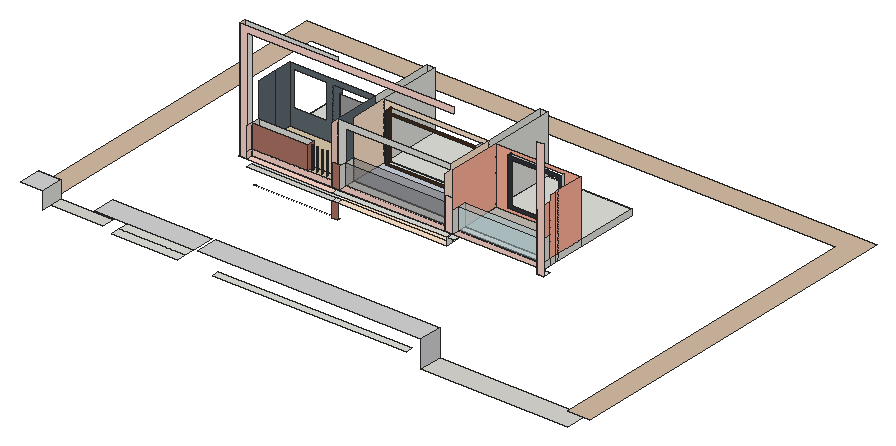
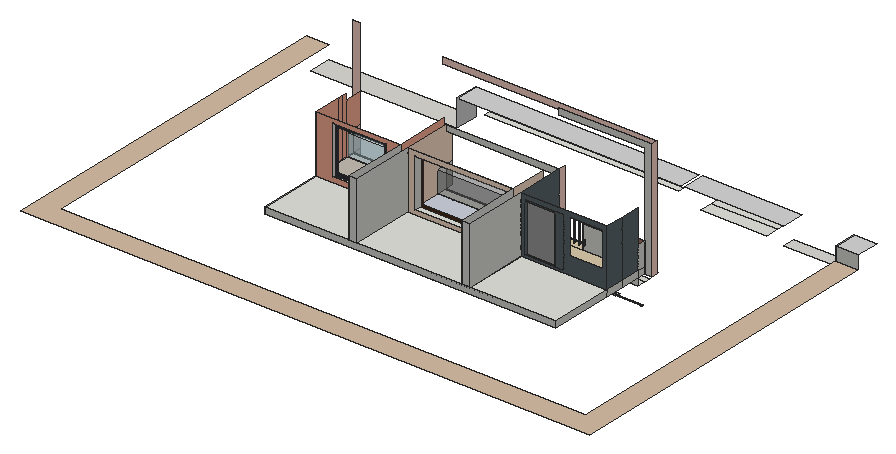
# SketchUp Ruby script. Lengths in inches.
U = 1.inch
M = Sketchup.active_model
def pt(a) = Geom::Point3d.new(a.map { |v| v * U })
def face(e, loops, mat)
  f = e.add_face(loops[0].map { |a| pt(a) })
  loops[1..].each { |l| e.add_face(l.map { |a| pt(a) }).erase! }
  f.material = f.back_material = mat if mat
  f
end
# faces: each face lists its corners as indices into pts; further lists are holes
def faces(e, pts, list, mat = nil) = list.each { |f| face(e, (f[0].is_a?(Array) ? f : [f]).map { |l| l.map { |i| pts[i] } }, mat) }
# xy, xz, yz: faces in a plane at the given z, y or x. An outline is a flat list of corners, or four numbers for a rectangle; further outlines are holes
def ring(l) = l.size == 4 ? [[l[0], l[1]], [l[2], l[1]], [l[2], l[3]], [l[0], l[3]]] : l.each_slice(2).to_a
def flat(e, list, mat, &to3) = list.each { |f| face(e, (f[0].is_a?(Array) ? f : [f]).map { |l| ring(l).map { |u, v| to3.(u, v) } }, mat) }
def xy(e, z, list, mat = nil) = flat(e, list, mat) { |x, y| [x, y, z] }
def xz(e, y, list, mat = nil) = flat(e, list, mat) { |x, z| [x, y, z] }
def yz(e, x, list, mat = nil) = flat(e, list, mat) { |y, z| [x, y, z] }
def lines(e, pts, list) = list.each { |a, b| e.add_line(pt(pts[a]), pt(pts[b])) }
# prism: a flat outline (further loops are holes) pulled along v
def prism(e, loops, v, mat = nil)
  f = face(e, loops, mat); d = Geom::Vector3d.new(v.map { |x| x * U })
  f.pushpull(f.normal.samedirection?(d) ? d.length : -d.length)
end
def box(e, o, s, mat = nil) = prism(e, [[o, [o[0] + s[0], o[1], o[2]], [o[0] + s[0], o[1] + s[1], o[2]], [o[0], o[1] + s[1], o[2]]]], [0, 0, s[2]], mat)
def at(x, y, z, deg = 0) = Geom::Transformation.translation(pt([x, y, z])) * Geom::Transformation.rotation(ORIGIN, Z_AXIS, deg.degrees)
def axes(o, x, y, z) = Geom::Transformation.new([*x, 0, *y, 0, *z, 0, *pt(o).to_a, 1])
def part(name) = M.definitions.add(name)
# library, detail: a bought-in or finely detailed component or shape, given as its bounding box
def library(name, o, s) = part(name).tap { |d| box(d.entities, o, s) }
def detail(e, o, s) = box(e.add_group.entities, o, s)
def put(e, d, t, mat = nil) = e.add_instance(d, t).tap { |i| i.material = mat if mat }
def group(e, t, mat = nil) = e.add_group.tap { |g| g.transformation = t; g.material = mat if mat }.entities
root = M.entities
M.materials.add("[Blinds Vertical Pattern]").color = [212, 212, 214]
M.materials.add("[Blinds Vertical Stripe Gray]").color = [160, 160, 160]
M.materials.add("[Color B01]").color = [255, 216, 204]
M.materials.add("[Color B02]").color = [255, 178, 153]
M.materials.add("[Color C01]").color = [255, 229, 204]
M.materials.add("[Field Rectangle Tile]").color = [196, 189, 179]
M.materials.add("[Field Square Tile]").color = [217, 201, 169]
M.materials.add("[Formica Graystone]").color = [149, 146, 135]
M.materials.add("[Formica Laminate Dark]").color = [50, 53, 60]
M.materials.add("[Formica Laminate Light]").color = [213, 189, 164]
M.materials.add("[Formica Speckled Grey]").color = [94, 105, 111]
M.materials.add("[Marble Carrara Floor Tile]").color = [204, 208, 219]
M.materials.add("[Stone Flagstone Ashlar]").color = [175, 116, 102]
M.materials.add("[Stone Flagstone Ashlar]1").color = [175, 116, 102]
M.materials.add("[Terrazzo Tile Light]").color = [219, 217, 210]
M.materials.add("[Translucent Glass Gray]").color = [128, 128, 128]
M.materials["[Translucent Glass Gray]"].alpha = 0.5
M.materials.add("[Translucent Glass Safety]").color = [204, 235, 244]
M.materials["[Translucent Glass Safety]"].alpha = 0.5
M.materials.add("[Wood Veneer 01]").color = [76, 44, 23]
xy(root,546.8125,[[2439.95,0,3329.24,137.64]],"[Terrazzo Tile Light]")
xy(root,604.375,[[137.64,62.625,453.55,137.64]],"[Terrazzo Tile Light]")
xy(root,610.51,[[1170.21,0,2349.69,42.1875]])
xy(root,619.23,[[1302.08,955.61,1426.75,983.36],[1442.97,955.61,1568.8125,983.36],[1585.03,955.61,1721.6875,983.36],[1737.9,955.61,1860.8,983.36]])
xy(root,623.51,[[554.87,0,956.3,58.3125],[554.87,58.3125,956.3,137.64]])
xy(root,631.3125,[[3329.24,0,3466.875,0,3466.875,2178.1875,0,2178.1875,0,137.64,137.64,137.64,137.64,2040.55,3329.24,2040.55]],"[Formica Laminate Light]")
xy(root,636.3125,[[1285,955.61,1877.875,983.36]],"[Wood Veneer 01]")
xy(root,642.77,[[914.91,1040.67,1175.1,1074.11]])
xy(root,646.07,[[723.26,1062.73,783.24,1074.11],[797.04,1062.73,861.24,1074.11]],"[Formica Speckled Grey]")
xy(root,657.36,[[1213.16,856.3125,1248.61,894.5]])
xy(root,657.36,[[1248.61,856.3125,1908.08,894.5],[1248.61,894.5,1908.08,950.43]],"[Color C01]")
xy(root,657.36,[[691.11,856.3125,1213.16,894.5],[691.11,894.5,1213.16,950.43]],"[Terrazzo Tile Light]")
xy(root,659.05,[[710.28,1062.73,874.22,1074.11]])
xy(root,659.56,[[2059.65,990.79,2174.84,1012.29],[2197.86,990.79,2308.19,1012.29]])
xy(root,672.85,[[2046.36,990.79,2321.48,1012.29]],"[Formica Laminate Dark]")
xy(root,702.75,[[2463.34,849.3125,2507.95,856.3125],[1213.16,856.3125,1908.08,894.5],[1908.08,856.3125,1953.74,899.87],[2463.34,856.3125,2507.95,894.5],[646.49,861.43,691.11,894.5],
  [646.49,894.5,691.11,899.87],[691.11,894.5,1213.16,899.87],[1213.16,894.5,1248.61,899.87],[1248.61,894.5,1908.08,899.87],[691.11,899.87,1213.16,950.43],
  [1213.16,899.87,1248.61,1126.61],[1248.61,899.87,1908.08,950.43],[1908.08,899.87,1938.3,1126.61],[1938.3,899.87,1953.74,1012.29],[691.11,950.43,1213.16,1074.11],
  [1248.61,950.43,1908.08,983.36],[1248.61,983.36,1248.61,1126.61,1213.16,1126.61,1213.16,1074.11,691.11,1074.11,691.11,1182.72,2463.34,1182.72,2463.34,1012.29,1938.3,1012.29,1938.3,1126.61,1908.08,1126.61,1908.08,983.36],[691.11,1182.72,2463.34,1571.68]])
xy(root,702.75,[[646.49,856.3125,1213.16,856.3125,1213.16,894.5,691.11,894.5,691.11,861.43,646.49,861.43]],"[Color B01]")
xy(root,702.75,[[1953.74,899.87,2463.34,1012.29]],"[Color B02]")
xy(root,712.1875,[[0,0,137.64,137.64],[453.55,0,1057.62,137.64],[1080.95,0,2439.95,137.64]],"[Blinds Vertical Pattern]")
xy(root,738.75,[[1214.63,849.3125,1263.92,894.5],[1905.54,849.3125,1950.59,899.87],[1214.63,894.5,1263.92,899.87],[1263.92,894.5,1905.54,899.87],[1950.59,894.5,2463.34,899.87],
  [691.11,899.87,1027.33,950.43],[1214.63,899.87,1263.92,1571.68],[1263.92,899.87,1905.54,954.56],[1905.54,899.87,1950.59,1571.68],[1950.59,899.87,2463.34,942.43],
  [1041.89,916.51,1040.81,916.65,1039.8,917.07,1038.93,917.73,1038.27,918.6,1037.85,919.61,1037.71,920.69,1037.85,921.78,1038.27,922.79,1038.93,923.65,1039.8,924.32,1040.81,924.74,1041.89,924.88,1042.98,924.74,1043.99,924.32,1044.85,923.65,1045.52,922.79,1045.9375,921.78,1046.08,920.69,1045.9375,919.61,1045.52,918.6,1044.85,917.73,1043.99,917.07,1042.98,916.65],[1070.77,916.51,1069.68,916.65,1068.67,917.07,1067.81,917.73,1067.14,918.6,1066.72,919.61,1066.58,920.69,1066.72,921.78,1067.14,922.79,1067.81,923.65,1068.67,924.32,1069.68,924.74,1070.77,924.88,1071.85,924.74,1072.86,924.32,1073.73,923.65,1074.39,922.79,1074.8125,921.78,1074.96,920.69,1074.8125,919.61,1074.39,918.6,1073.73,917.73,1072.86,917.07,1071.85,916.65],[1101.58,916.51,1100.5,916.65,1099.49,917.07,1098.62,917.73,1097.95,918.6,1097.54,919.61,1097.39,920.69,1097.54,921.78,1097.95,922.79,1098.62,923.65,1099.49,924.32,1100.5,924.74,1101.58,924.88,1102.66,924.74,1103.67,924.32,1104.54,923.65,1105.21,922.79,1105.625,921.78,1105.77,920.69,1105.625,919.61,1105.21,918.6,1104.54,917.73,1103.67,917.07,1102.66,916.65],[1131.83,916.51,1130.75,916.65,1129.74,917.07,1128.87,917.73,1128.2,918.6,1127.79,919.61,1127.64,920.69,1127.79,921.78,1128.2,922.79,1128.87,923.65,1129.74,924.32,1130.75,924.74,1131.83,924.88,1132.91,924.74,1133.92,924.32,1134.79,923.65,1135.46,922.79,1135.875,921.78,1136.02,920.69,1135.875,919.61,1135.46,918.6,1134.79,917.73,1133.92,917.07,1132.91,916.65],[1167.14,916.51,1166.06,916.65,1165.05,917.07,1164.18,917.73,1163.52,918.6,1163.1,919.61,1162.96,920.69,1163.1,921.78,1163.52,922.79,1164.18,923.65,1165.05,924.32,1166.06,924.74,1167.14,924.88,1168.23,924.74,1169.24,924.32,1170.1,923.65,1170.77,922.79,1171.1875,921.78,1171.33,920.69,1171.1875,919.61,1170.77,918.6,1170.1,917.73,1169.24,917.07,1168.23,916.65],
  [1198.52,916.51,1197.43,916.65,1196.42,917.07,1195.56,917.73,1194.89,918.6,1194.47,919.61,1194.33,920.69,1194.47,921.78,1194.89,922.79,1195.56,923.65,1196.42,924.32,1197.43,924.74,1198.52,924.88,1199.6,924.74,1200.61,924.32,1201.48,923.65,1202.14,922.79,1202.5625,921.78,1202.71,920.69,1202.5625,919.61,1202.14,918.6,1201.48,917.73,1200.61,917.07,1199.6,916.65],[691.11,1182.72,1214.63,1571.68],[1263.92,1182.72,1905.54,1571.68],[1950.59,1182.72,2463.34,1571.68]])
xy(root,738.75,[[1950.59,942.43,2463.34,1182.72]],"[Field Rectangle Tile]")
xy(root,738.75,[[[1027.33,899.87,1214.63,950.43],[1041.89,916.51,1040.81,916.65,1039.8,917.07,1038.93,917.73,1038.27,918.6,1037.85,919.61,1037.71,920.69,1037.85,921.78,1038.27,922.79,1038.93,923.65,1039.8,924.32,1040.81,924.74,1041.89,924.88,1042.98,924.74,1043.99,924.32,1044.85,923.65,1045.52,922.79,1045.9375,921.78,1046.08,920.69,1045.9375,919.61,1045.52,918.6,1044.85,917.73,1043.99,917.07,1042.98,916.65],[1198.52,916.51,1197.43,916.65,1196.42,917.07,1195.56,917.73,1194.89,918.6,1194.47,919.61,1194.33,920.69,1194.47,921.78,1194.89,922.79,1195.56,923.65,1196.42,924.32,1197.43,924.74,1198.52,924.88,1199.6,924.74,1200.61,924.32,1201.48,923.65,1202.14,922.79,1202.5625,921.78,1202.71,920.69,1202.5625,919.61,1202.14,918.6,1201.48,917.73,1200.61,917.07,1199.6,916.65],[1070.77,916.51,1069.68,916.65,1068.67,917.07,1067.81,917.73,1067.14,918.6,1066.72,919.61,1066.58,920.69,1066.72,921.78,1067.14,922.79,1067.81,923.65,1068.67,924.32,1069.68,924.74,1070.77,924.88,1071.85,924.74,1072.86,924.32,1073.73,923.65,1074.39,922.79,1074.8125,921.78,1074.96,920.69,1074.8125,919.61,1074.39,918.6,1073.73,917.73,1072.86,917.07,1071.85,916.65],[1167.14,916.51,1166.06,916.65,1165.05,917.07,1164.18,917.73,1163.52,918.6,1163.1,919.61,1162.96,920.69,1163.1,921.78,1163.52,922.79,1164.18,923.65,1165.05,924.32,1166.06,924.74,1167.14,924.88,1168.23,924.74,1169.24,924.32,1170.1,923.65,1170.77,922.79,1171.1875,921.78,1171.33,920.69,1171.1875,919.61,1170.77,918.6,1170.1,917.73,1169.24,917.07,1168.23,916.65],[1101.58,916.51,1100.5,916.65,1099.49,917.07,1098.62,917.73,1097.95,918.6,1097.54,919.61,1097.39,920.69,1097.54,921.78,1097.95,922.79,1098.62,923.65,1099.49,924.32,1100.5,924.74,1101.58,924.88,1102.66,924.74,1103.67,924.32,1104.54,923.65,1105.21,922.79,1105.625,921.78,1105.77,920.69,1105.625,919.61,1105.21,918.6,1104.54,917.73,1103.67,917.07,1102.66,916.65],[1131.83,916.51,1130.75,916.65,1129.74,917.07,1128.87,917.73,1128.2,918.6,1127.79,919.61,1127.64,920.69,1127.79,921.78,1128.2,922.79,1128.87,923.65,1129.74,924.32,1130.75,924.74,1131.83,924.88,1132.91,924.74,1133.92,924.32,1134.79,923.65,1135.46,922.79,1135.875,921.78,1136.02,920.69,1135.875,919.61,1135.46,918.6,1134.79,917.73,1133.92,917.07,1132.91,916.65]],[691.11,950.43,1214.63,1182.72]],"[Field Square Tile]")
xy(root,738.75,[[1263.92,954.56,1905.54,1182.72]],"[Marble Carrara Floor Tile]")
xy(root,750.91,[[1009.02,1166.28,1195.59,1182.72]])
xy(root,762.1,[[1310.9,1141.09,1861.28,1182.72]])
xy(root,769.59,[[2036.23,1166.78,2361.3,1182.72]])
xz(root,137.64,[[0,631.3125,137.64,712.1875]])
xz(root,849.3125,[[2463.34,702.75,2507.95,1424.1875],[1905.54,738.75,1950.59,937.95]],"[Color B01]")
xz(root,849.3125,[[1214.63,738.75,1263.92,872.4]],"[Stone Flagstone Ashlar]1")
xz(root,856.3125,[[1213.16,566.24,1248.61,657.36]],"[Stone Flagstone Ashlar]1")
xz(root,861.43,[[646.49,702.75,691.11,702.75,691.11,1387.1,1950.59,1387.1,1950.59,1424.1875,646.49,1424.1875]],"[Color B01]")
xz(root,894.5,[[1214.63,738.75,1214.63,1086.8125,1905.54,1086.8125,1905.54,1051.41,1263.92,1051.41,1263.92,738.75]])
xz(root,894.5,[[1263.92,738.75,1905.54,868.4375]],"[Translucent Glass Gray]")
xz(root,894.5,[[1950.59,738.75,2463.34,868.4375]],"[Translucent Glass Safety]")
xz(root,899.87,[[646.49,702.75,646.49,1424.1875,1214.63,1424.1875,1214.63,1387.1,691.11,1387.1,691.11,702.75]])
xz(root,899.87,[[691.11,702.75,2463.34,738.75]],"[Color B01]")
xz(root,899.87,[[691.11,738.75,1027.33,880]],"[Stone Flagstone Ashlar]")
xz(root,942.43,[[1950.59,738.75,2463.34,868.4375]],"[Translucent Glass Safety]")
xz(root,950.43,[[691.11,657.36,1213.16,702.75],[1248.61,657.36,1908.08,702.75],[691.11,738.75,1027.33,880]])
xz(root,954.56,[[1263.92,738.75,1905.54,868.4375]],"[Translucent Glass Gray]")
xz(root,1141.09,[[[1310.9,762.1,1861.28,1059.16],[1324.98,776.18,1847.2,1045.08]]],"[Wood Veneer 01]")
xz(root,1166.28,[[1009.02,750.91,1195.59,1033.9]],"[Blinds Vertical Stripe Gray]")
xz(root,1166.78,[[[2036.23,769.59,2361.3,1063.34],[2056.09,789.44,2341.44,1043.49]]],"[Formica Laminate Dark]")
xz(root,1182.72,[[[1950.59,738.75,2463.34,1086.8125],[2036.23,769.59,2361.3,1063.34]]],"[Color B02]")
xz(root,1182.72,[[[1263.92,738.75,1905.54,1086.8125],[1310.9,762.1,1861.28,1059.16]]],"[Color C01]")
xz(root,1182.72,[[[691.11,738.75,1214.63,1086.8125],[955.69,750.91,955.69,1058.91,917.47,1058.91,917.47,844.43,715.78,844.43,715.78,1058.91,1195.59,1058.91,1195.59,750.91]],[955.69,750.91,1009.02,1058.91]],"[Formica Speckled Grey]")
xz(root,1571.68,[[691.11,702.75,2463.34,738.75],[1214.63,738.75,1263.92,1086.8125],[1905.54,738.75,1950.59,1086.8125]])
yz(root,137.64,[[0,604.375,137.64,712.1875]])
yz(root,646.49,[[861.43,702.75,899.87,1424.1875]],"[Color B01]")
yz(root,691.11,[[899.87,702.75,950.43,738.75],[950.43,702.75,1074.11,738.75],[1074.11,702.75,1182.72,738.75],[1182.72,702.75,1571.68,738.75],[899.87,738.75,950.43,880]])
yz(root,691.11,[[861.43,702.75,899.87,738.75],[861.43,738.75,899.87,880]],"[Color B01]")
yz(root,691.11,[[950.43,738.75,1074.11,1086.8125],[1074.11,738.75,1182.72,1086.8125]],"[Formica Speckled Grey]")
yz(root,1009.02,[[1166.28,750.91,1182.72,1033.9]],"[Formica Speckled Grey]")
yz(root,1027.33,[[[899.87,738.75,950.43,880],[922.52,862.65,921.05,862.84,919.68,863.41,918.5,864.32,917.6,865.49,917.03,866.87,916.84,868.34,917.03,869.81,917.6,871.18,918.5,872.36,919.68,873.26,921.05,873.83,922.52,874.02,923.99,873.83,925.37,873.26,926.54,872.36,927.45,871.18,928.02,869.81,928.21,868.34,928.02,866.87,927.45,865.49,926.54,864.32,925.37,863.41,923.99,862.84]]],"[Stone Flagstone Ashlar]")
yz(root,1195.59,[[1166.28,750.91,1182.72,1033.9]],"[Formica Speckled Grey]")
yz(root,1214.63,[[1182.72,738.75,1571.68,1086.8125]])
yz(root,1214.63,[[849.3125,738.75,894.5,1086.8125]],"[Color B01]")
yz(root,1214.63,[[[894.5,738.75,1182.72,1086.8125],[922.52,862.65,923.99,862.84,925.37,863.41,926.54,864.32,927.45,865.49,928.02,866.87,928.21,868.34,928.02,869.81,927.45,871.18,926.54,872.36,925.37,873.26,923.99,873.83,922.52,874.02,921.05,873.83,919.68,873.26,918.5,872.36,917.6,871.18,917.03,869.81,916.84,868.34,917.03,866.87,917.6,865.49,918.5,864.32,919.68,863.41,921.05,862.84]]],"[Formica Speckled Grey]")
yz(root,1263.92,[[849.3125,738.75,894.5,868.4375],[894.5,738.75,954.56,868.4375],[1182.72,738.75,1571.68,1086.8125]])
yz(root,1263.92,[[954.56,738.75,1182.72,1086.8125]],"[Color C01]")
yz(root,1310.9,[[1141.09,762.1,1182.72,1059.16]],"[Wood Veneer 01]")
yz(root,1861.28,[[1141.09,762.1,1182.72,1059.16]])
yz(root,1905.54,[[849.3125,738.75,894.5,868.4375],[894.5,738.75,954.56,868.4375],[1182.72,738.75,1571.68,1086.8125]])
yz(root,1905.54,[[[954.56,738.75,954.56,868.4375,849.3125,868.4375,849.3125,1051.41,894.5,1051.41,894.5,1086.8125,1182.72,1086.8125,1182.72,738.75],[923.73,877.96,925.46,878.18,927.08,878.85,928.46,879.91,929.52,881.3,930.19,882.91,930.42,884.64,930.19,886.375,929.52,887.99,928.46,889.37,927.08,890.43,925.46,891.1,923.73,891.33,922,891.1,920.39,890.43,919,889.37,917.94,887.99,917.27,886.375,917.04,884.64,917.27,882.91,917.94,881.3,919,879.91,920.39,878.85,922,878.18]]],"[Color C01]")
yz(root,1908.08,[[856.3125,657.36,894.5,702.75]])
yz(root,1950.59,[[849.3125,738.75,894.5,868.4375],[894.5,738.75,942.43,868.4375],[1182.72,738.75,1571.68,1086.8125]])
yz(root,1950.59,[[[942.43,738.75,1182.72,738.75,1182.72,1086.8125,849.3125,1086.8125,849.3125,868.4375,942.43,868.4375],[918.47,876.58,917.1875,876.75,916,877.24,914.97,878.03,914.1875,879.05,913.7,880.24,913.53,881.52,913.7,882.8,914.1875,883.99,914.97,885.01,916,885.8,917.1875,886.29,918.47,886.46,919.74,886.29,920.93,885.8,921.96,885.01,922.74,883.99,923.23,882.8,923.4,881.52,923.23,880.24,922.74,879.05,921.96,878.03,920.93,877.24,919.74,876.75]]],"[Color B02]")
yz(root,2036.23,[[1166.78,769.59,1182.72,1063.34]],"[Formica Laminate Dark]")
yz(root,2361.3,[[1166.78,769.59,1182.72,1063.34]])
yz(root,2439.95,[[0,546.8125,137.64,712.1875]],"[Blinds Vertical Pattern]")
yz(root,2463.34,[[899.87,702.75,950.43,738.75],[950.43,702.75,983.36,738.75],[983.36,702.75,1012.29,738.75],[1012.29,702.75,1182.72,738.75],[1182.72,702.75,1571.68,738.75],
  [894.5,738.75,942.43,868.4375]])
yz(root,2463.34,[[849.3125,702.75,899.87,738.75],[849.3125,738.75,894.5,868.4375]],"[Color B01]")
yz(root,2463.34,[[[942.43,738.75,942.43,868.4375,849.3125,868.4375,849.3125,1051.41,950.43,1051.41,950.43,738.75],[918.47,876.58,919.74,876.75,920.93,877.24,921.96,878.03,922.74,879.05,923.23,880.24,923.4,881.52,923.23,882.8,922.74,883.99,921.96,885.01,920.93,885.8,919.74,886.29,918.47,886.46,917.1875,886.29,916,885.8,914.97,885.01,914.1875,883.99,913.7,882.8,913.53,881.52,913.7,880.24,914.1875,879.05,914.97,878.03,916,877.24,917.1875,876.75]],[950.43,738.75,950.43,1051.41,954.56,1051.41,954.56,1086.8125,983.36,1086.8125,983.36,738.75],[983.36,738.75,1012.29,1086.8125],[1012.29,738.75,1182.72,1086.8125]],"[Color B02]")
p = [[1213.16,911.02,535.46],[1213.16,911.77,536.03],[691.11,911.77,536.03],[691.11,911.02,535.46],[1213.16,915.37,536.03],[1213.16,916.11,535.46],
  [691.11,916.11,535.46],[691.11,915.37,536.03],[1213.16,912.64,536.39],[691.11,912.64,536.39],[1213.16,914.5,536.39],[691.11,914.5,536.39],
  [1213.16,913.57,536.52],[691.11,913.57,536.52],[1040.81,916.65,738.75],[1041.89,916.51,738.75],[1041.89,916.51,871.5625],[1040.81,916.65,871.5625],
  [1042.98,916.65,738.75],[1042.98,916.65,871.5625],[1069.68,916.65,738.75],[1070.77,916.51,738.75],[1070.77,916.51,871.18],[1069.68,916.65,871.18],
  [1071.85,916.65,738.75],[1071.85,916.65,871.18],[1100.5,916.65,738.75],[1101.58,916.51,738.75],[1101.58,916.51,868.5625],[1100.5,916.65,868.5625],
  [1102.66,916.65,738.75],[1102.66,916.65,868.5625],[1130.75,916.65,738.75],[1131.83,916.51,738.75],[1131.83,916.51,868.4375],[1130.75,916.65,868.4375],
  [1132.91,916.65,738.75],[1132.91,916.65,868.4375],[1166.06,916.65,738.75],[1167.14,916.51,738.75],[1167.14,916.51,868.875],[1166.06,916.65,868.875],
  [1168.23,916.65,738.75],[1168.23,916.65,868.875],[1197.43,916.65,738.75],[1198.52,916.51,738.75],[1198.52,916.51,869.875],[1197.43,916.65,869.875],
  [1199.6,916.65,738.75],[1199.6,916.65,869.875],[1039.8,917.07,738.75],[1039.8,917.07,871.5625],[1043.99,917.07,738.75],[1043.99,917.07,871.5625],
  [1068.67,917.07,738.75],[1068.67,917.07,871.18],[1072.86,917.07,738.75],[1072.86,917.07,871.18],[1099.49,917.07,738.75],[1099.49,917.07,868.5625],
  [1103.67,917.07,738.75],[1103.67,917.07,868.5625],[1129.74,917.07,738.75],[1129.74,917.07,868.4375],[1133.92,917.07,738.75],[1133.92,917.07,868.4375],
  [1165.05,917.07,738.75],[1165.05,917.07,868.875],[1169.24,917.07,738.75],[1169.24,917.07,868.875],[1196.42,917.07,738.75],[1196.42,917.07,869.875],
  [1200.61,917.07,738.75],[1200.61,917.07,869.875],[1038.93,917.73,738.75],[1038.93,917.73,871.5625],[1044.85,917.73,738.75],[1044.85,917.73,871.5625],
  [1067.81,917.73,738.75],[1067.98,917.6,871.18],[1067.81,917.73,871.18],[1073.73,917.73,738.75],[1073.73,917.73,871.18],[1073.55,917.6,871.18],
  [1098.62,917.73,738.75],[1098.62,917.73,868.5625],[1104.54,917.73,738.75],[1104.54,917.73,868.5625],[1128.87,917.73,738.75],[1128.87,917.73,868.4375],
  [1134.79,917.73,738.75],[1134.79,917.73,868.4375],[1164.18,917.73,738.75],[1164.18,917.73,868.875],[1170.1,917.73,738.75],[1170.1,917.73,868.875],
  [1195.56,917.73,738.75],[1195.56,917.73,869.875],[1201.48,917.73,738.75],[1201.48,917.73,869.875],[1038.27,918.6,738.75],[1038.27,918.6,871.5625],
  [1045.52,918.6,738.75],[1045.52,918.6,871.5625],[1067.14,918.6,738.75],[1067.14,918.6,871.18],[1074.39,918.6,738.75],[1074.39,918.6,871.18],
  [1097.95,918.6,738.75],[1097.95,918.6,868.5625],[1105.21,918.6,738.75],[1105.21,918.6,868.5625],[1128.2,918.6,738.75],[1128.2,918.6,868.4375],
  [1135.46,918.6,738.75],[1135.46,918.6,868.4375],[1163.52,918.6,738.75],[1163.52,918.6,868.875],[1170.77,918.6,738.75],[1170.77,918.6,868.875],
  [1194.89,918.6,738.75],[1194.89,918.6,869.875],[1202.14,918.6,738.75],[1202.14,918.6,869.875],[1037.85,919.61,738.75],[1037.85,919.61,871.5625],
  [1045.9375,919.61,738.75],[1045.9375,919.61,871.5625],[1066.72,919.61,738.75],[1066.72,919.61,871.18],[1074.8125,919.61,738.75],[1074.8125,919.61,871.18],
  [1097.54,919.61,738.75],[1097.54,919.61,868.5625],[1105.625,919.61,738.75],[1105.625,919.61,868.5625],[1127.79,919.61,738.75],[1127.79,919.61,868.4375],
  [1135.875,919.61,738.75],[1135.875,919.61,868.4375],[1163.1,919.61,738.75],[1163.1,919.61,868.875],[1171.1875,919.61,738.75],[1171.1875,919.61,868.875],
  [1194.47,919.61,738.75],[1194.47,919.61,869.875],[1202.5625,919.61,738.75],[1202.5625,919.61,869.875],[1037.71,920.69,738.75],[1037.71,920.69,871.5625],
  [1046.08,920.69,738.75],[1046.08,920.69,871.5625],[1066.58,920.69,738.75],[1066.58,920.69,871.18],[1074.96,920.69,738.75],[1074.96,920.69,871.18],
  [1097.39,920.69,738.75],[1097.39,920.69,868.5625],[1105.77,920.69,738.75],[1105.77,920.69,868.5625],[1127.64,920.69,738.75],[1127.64,920.69,868.4375],
  [1136.02,920.69,738.75],[1136.02,920.69,868.4375],[1162.96,920.69,738.75],[1162.96,920.69,868.875],[1171.33,920.69,738.75],[1171.33,920.69,868.875],
  [1194.33,920.69,738.75],[1194.33,920.69,869.875],[1202.71,920.69,738.75],[1202.71,920.69,869.875],[1037.85,921.78,738.75],[1037.85,921.78,871.5625],
  [1045.9375,921.78,738.75],[1045.9375,921.78,871.5625],[1066.72,921.78,738.75],[1066.72,921.78,871.18],[1074.8125,921.78,738.75],[1074.8125,921.78,871.18],
  [1097.54,921.78,738.75],[1097.54,921.78,868.5625],[1105.625,921.78,738.75],[1105.625,921.78,868.5625],[1127.79,921.78,738.75],[1127.79,921.78,868.4375],
  [1135.875,921.78,738.75],[1135.875,921.78,868.4375],[1163.1,921.78,738.75],[1163.1,921.78,868.875],[1171.1875,921.78,738.75],[1171.1875,921.78,868.875],
  [1194.47,921.78,738.75],[1194.47,921.78,869.875],[1202.5625,921.78,738.75],[1202.5625,921.78,869.875],[1038.27,922.79,738.75],[1038.27,922.79,871.5625],
  [1045.52,922.79,738.75],[1045.52,922.79,871.5625],[1067.14,922.79,738.75],[1067.14,922.79,871.18],[1074.39,922.79,738.75],[1074.39,922.79,871.18],
  [1097.95,922.79,738.75],[1097.95,922.79,868.5625],[1105.21,922.79,738.75],[1105.21,922.79,868.5625],[1128.2,922.79,738.75],[1128.2,922.79,868.4375],
  [1135.46,922.79,738.75],[1135.46,922.79,868.4375],[1163.52,922.79,738.75],[1163.52,922.79,868.875],[1170.77,922.79,738.75],[1170.77,922.79,868.875],
  [1194.89,922.79,738.75],[1194.89,922.79,869.875],[1202.14,922.79,738.75],[1202.14,922.79,869.875],[1038.93,923.65,738.75],[1038.93,923.65,871.5625],
  [1044.85,923.65,738.75],[1044.85,923.65,871.5625],[1067.81,923.65,738.75],[1067.81,923.65,871.18],[1073.73,923.65,738.75],[1073.73,923.65,871.18],
  [1098.62,923.65,738.75],[1098.62,923.65,868.5625],[1104.54,923.65,738.75],[1104.54,923.65,868.5625],[1128.87,923.65,738.75],[1128.87,923.65,868.4375],
  [1134.79,923.65,738.75],[1134.79,923.65,868.4375],[1164.18,923.65,738.75],[1164.18,923.65,868.875],[1170.1,923.65,738.75],[1170.1,923.65,868.875],
  [1195.56,923.65,738.75],[1195.56,923.65,869.875],[1201.48,923.65,738.75],[1201.48,923.65,869.875],[1039.8,924.32,738.75],[1039.8,924.32,871.5625],
  [1043.99,924.32,738.75],[1043.99,924.32,871.5625],[1068.67,924.32,738.75],[1068.67,924.32,871.18],[1072.86,924.32,738.75],[1072.86,924.32,871.18],
  [1099.49,924.32,738.75],[1099.49,924.32,868.5625],[1103.67,924.32,738.75],[1103.67,924.32,868.5625],[1129.74,924.32,738.75],[1129.74,924.32,868.4375],
  [1133.92,924.32,738.75],[1133.92,924.32,868.4375],[1165.05,924.32,738.75],[1165.05,924.32,868.875],[1169.24,924.32,738.75],[1169.24,924.32,868.875],
  [1196.42,924.32,738.75],[1196.42,924.32,869.875],[1200.61,924.32,738.75],[1200.61,924.32,869.875],[1040.81,924.74,738.75],[1040.81,924.74,871.5625],
  [1042.98,924.74,738.75],[1042.98,924.74,871.5625],[1069.68,924.74,738.75],[1069.68,924.74,871.18],[1071.85,924.74,738.75],[1071.85,924.74,871.18],
  [1100.5,924.74,738.75],[1100.5,924.74,868.5625],[1102.66,924.74,738.75],[1102.66,924.74,868.5625],[1130.75,924.74,738.75],[1130.75,924.74,868.4375],
  [1132.91,924.74,738.75],[1132.91,924.74,868.4375],[1166.06,924.74,738.75],[1166.06,924.74,868.875],[1168.23,924.74,738.75],[1168.23,924.74,868.875],
  [1197.43,924.74,738.75],[1197.43,924.74,869.875],[1199.6,924.74,738.75],[1199.6,924.74,869.875],[1041.89,924.88,738.75],[1041.89,924.88,871.5625],
  [1070.77,924.88,738.75],[1070.77,924.88,871.18],[1101.58,924.88,738.75],[1101.58,924.88,868.5625],[1131.83,924.88,738.75],[1131.83,924.88,868.4375],
  [1167.14,924.88,738.75],[1167.14,924.88,868.875],[1198.52,924.88,738.75],[1198.52,924.88,869.875]]
faces(root,p,[[0,1,2,3],[4,5,6,7],[1,8,9,2],[10,4,7,11],[8,12,13,9],[12,10,11,13]],"[Formica Laminate Dark]")
faces(root,p,[[14,15,16,17],[15,18,19,16],[20,21,22,23],[21,24,25,22],[26,27,28,29],[27,30,31,28],[32,33,34,35],[33,36,37,34],
  [38,39,40,41],[39,42,43,40],[44,45,46,47],[45,48,49,46],[50,14,17,51],[18,52,53,19],[54,20,23,55],[24,56,57,25],
  [58,26,29,59],[30,60,61,31],[62,32,35,63],[36,64,65,37],[66,38,41,67],[42,68,69,43],[70,44,47,71],[48,72,73,49],
  [74,50,51,75],[52,76,77,53],[78,54,55,79,80],[56,81,82,83,57],[84,58,59,85],[60,86,87,61],[88,62,63,89],[64,90,91,65],
  [92,66,67,93],[68,94,95,69],[96,70,71,97],[72,98,99,73],[100,74,75,101],[76,102,103,77],[104,78,80,105],[81,106,107,82],
  [108,84,85,109],[86,110,111,87],[112,88,89,113],[90,114,115,91],[116,92,93,117],[94,118,119,95],[120,96,97,121],[98,122,123,99],
  [124,100,101,125],[102,126,127,103],[128,104,105,129],[106,130,131,107],[132,108,109,133],[110,134,135,111],[136,112,113,137],[114,138,139,115],
  [140,116,117,141],[118,142,143,119],[144,120,121,145],[122,146,147,123],[148,124,125,149],[126,150,151,127],[152,128,129,153],[130,154,155,131],
  [156,132,133,157],[134,158,159,135],[160,136,137,161],[138,162,163,139],[164,140,141,165],[142,166,167,143],[168,144,145,169],[146,170,171,147],
  [172,148,149,173],[150,174,175,151],[176,152,153,177],[154,178,179,155],[180,156,157,181],[158,182,183,159],[184,160,161,185],[162,186,187,163],
  [188,164,165,189],[166,190,191,167],[192,168,169,193],[170,194,195,171],[196,172,173,197],[174,198,199,175],[200,176,177,201],[178,202,203,179],
  [204,180,181,205],[182,206,207,183],[208,184,185,209],[186,210,211,187],[212,188,189,213],[190,214,215,191],[216,192,193,217],[194,218,219,195],
  [220,196,197,221],[198,222,223,199],[224,200,201,225],[202,226,227,203],[228,204,205,229],[206,230,231,207],[232,208,209,233],[210,234,235,211],
  [236,212,213,237],[214,238,239,215],[240,216,217,241],[218,242,243,219],[244,220,221,245],[222,246,247,223],[248,224,225,249],[226,250,251,227],
  [252,228,229,253],[230,254,255,231],[256,232,233,257],[234,258,259,235],[260,236,237,261],[238,262,263,239],[264,240,241,265],[242,266,267,243],
  [268,244,245,269],[246,270,271,247],[272,248,249,273],[250,274,275,251],[276,252,253,277],[254,278,279,255],[280,256,257,281],[258,282,283,259],
  [284,260,261,285],[262,286,287,263],[288,264,265,289],[266,290,291,267],[292,268,269,293],[270,292,293,271],[294,272,273,295],[274,294,295,275],
  [296,276,277,297],[278,296,297,279],[298,280,281,299],[282,298,299,283],[300,284,285,301],[286,300,301,287],[302,288,289,303],[290,302,303,291]],"[Formica Graystone]")
